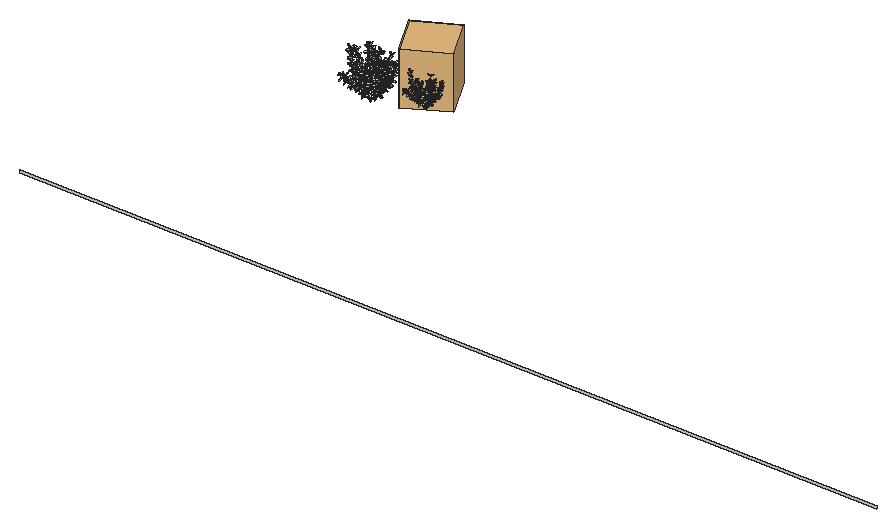
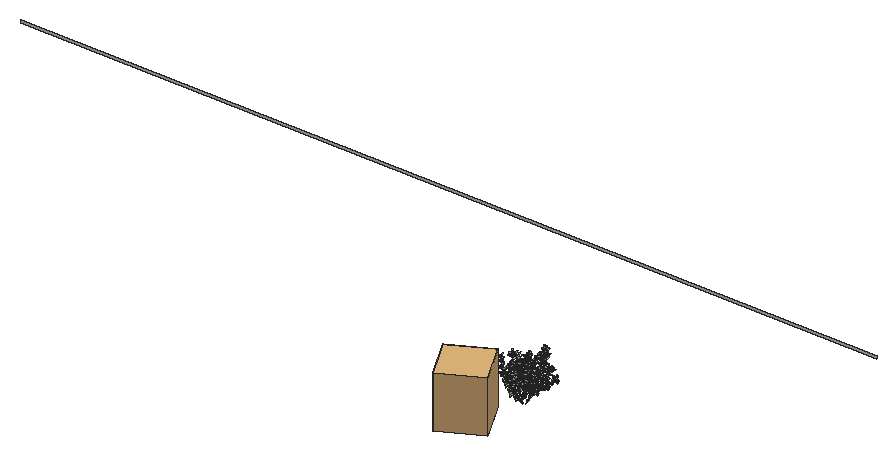
# SketchUp Ruby script. Lengths in inches.
U = 1.inch
M = Sketchup.active_model
def pt(a) = Geom::Point3d.new(a.map { |v| v * U })
def face(e, loops, mat)
  f = e.add_face(loops[0].map { |a| pt(a) })
  loops[1..].each { |l| e.add_face(l.map { |a| pt(a) }).erase! }
  f.material = f.back_material = mat if mat
  f
end
# faces: each face lists its corners as indices into pts; further lists are holes
def faces(e, pts, list, mat = nil) = list.each { |f| face(e, (f[0].is_a?(Array) ? f : [f]).map { |l| l.map { |i| pts[i] } }, mat) }
# xy, xz, yz: faces in a plane at the given z, y or x. An outline is a flat list of corners, or four numbers for a rectangle; further outlines are holes
def ring(l) = l.size == 4 ? [[l[0], l[1]], [l[2], l[1]], [l[2], l[3]], [l[0], l[3]]] : l.each_slice(2).to_a
def flat(e, list, mat, &to3) = list.each { |f| face(e, (f[0].is_a?(Array) ? f : [f]).map { |l| ring(l).map { |u, v| to3.(u, v) } }, mat) }
def xy(e, z, list, mat = nil) = flat(e, list, mat) { |x, y| [x, y, z] }
def xz(e, y, list, mat = nil) = flat(e, list, mat) { |x, z| [x, y, z] }
def yz(e, x, list, mat = nil) = flat(e, list, mat) { |y, z| [x, y, z] }
def lines(e, pts, list) = list.each { |a, b| e.add_line(pt(pts[a]), pt(pts[b])) }
# prism: a flat outline (further loops are holes) pulled along v
def prism(e, loops, v, mat = nil)
  f = face(e, loops, mat); d = Geom::Vector3d.new(v.map { |x| x * U })
  f.pushpull(f.normal.samedirection?(d) ? d.length : -d.length)
end
def box(e, o, s, mat = nil) = prism(e, [[o, [o[0] + s[0], o[1], o[2]], [o[0] + s[0], o[1] + s[1], o[2]], [o[0], o[1] + s[1], o[2]]]], [0, 0, s[2]], mat)
def at(x, y, z, deg = 0) = Geom::Transformation.translation(pt([x, y, z])) * Geom::Transformation.rotation(ORIGIN, Z_AXIS, deg.degrees)
def axes(o, x, y, z) = Geom::Transformation.new([*x, 0, *y, 0, *z, 0, *pt(o).to_a, 1])
def part(name) = M.definitions.add(name)
# library, detail: a bought-in or finely detailed component or shape, given as its bounding box
def library(name, o, s) = part(name).tap { |d| box(d.entities, o, s) }
def detail(e, o, s) = box(e.add_group.entities, o, s)
def put(e, d, t, mat = nil) = e.add_instance(d, t).tap { |i| i.material = mat if mat }
def group(e, t, mat = nil) = e.add_group.tap { |g| g.transformation = t; g.material = mat if mat }.entities
root = M.entities
M.materials.add("0ad16as01f6asdLeafVar1sfd015as60f1as6").color = [231, 235, 211]
M.materials.add("asdfasdf0165f6asdLeafVar1sfd015as60f1as6").color = [231, 235, 211]
M.materials.add("dw_stemssadfasdfa0sdf1s01d6w1").color = [90, 97, 50]
c1 = part("vdw_leaf\#1")
p = [[0,0,0],[-2.77,1.61,2.32],[-4.3125,6.1,4.5],[-3.97,13.49,6.09],[-2.47,18.57,6.3],[-0.2,22.73,5.75],
  [2.54,19.66,6.85],[4.3,15.93,7.09],[5.03,7.6,5.43],[3.32,1.76,2.74]]
faces(c1.entities,p,[[0,1,2,3,4,5],[0,5,6,7,8,9]],"0ad16as01f6asdLeafVar1sfd015as60f1as6")
c2 = part("dw_branch_3\#2")
p = [[-10.06,-1.6,62.9],[-0.2,1.54,-0.01],[-10.43,1.54,62.72],[0.18,-1.6,0.17],[-23.75,-21.66,88.91],[-25.7,-20.3,89.55],
  [13.4,11.62,104.56],[13.33,13.52,104.47],[-49.25,-41.87,130.3125],[-50.33,-40.21,130.71],[-4.97,21.13,143.98],[35.61,27.99,178.64],
  [-5.09,23.64,143.96],[35.32,29.14,178.46],[-67.7,-55.38,181.06],[-68.34,-54.45,181.62],[-22.8125,33.9,200.59],[-22.94,35.79,200.41],
  [56.61,36.78,229.75],[56.29,38.09,229.57],[-70.63,-67.46,248.85],[-70.72,-66.33,249.5],[-25.05,43.32,240.75],[-24.98,44.26,240.57]]
faces(c2.entities,p,[[0,1,2],[0,3,1],[4,2,5],[4,0,2],[6,0,2],[6,2,7],[8,4,5],[8,5,9],
  [10,6,7],[11,6,7],[10,7,12],[11,7,13],[14,8,9],[14,9,15],[16,10,12],[16,12,17],
  [18,11,13],[18,13,19],[20,14,15],[20,15,21],[22,16,17],[22,17,23]],"dw_stemssadfasdfa0sdf1s01d6w1")
c3 = part("dw_branch3\#2")
put(c3.entities,c1,axes([-70.33,-63.58,233.32],[-1.00752,0.412,0.78596],[-0.24851,-1.22189,0.32195],[0.83141,0.09817,1.01433]))
put(c3.entities,c1,axes([-66.93,-54.91,182.82],[-0.84976,-0.98359,0.33619],[0.99572,-0.74889,0.32577],[-0.05223,0.46521,1.22907]))
put(c3.entities,c1,axes([-46.12,-39.49,126.35],[1.23843,0.5364,0.23552],[-0.56438,0.94474,0.81599],[0.15707,-0.83465,1.07498]))
put(c3.entities,c1,axes([13.0625,13.13,104.77],[-1.01271,0.69982,-0.26884],[-0.74268,-0.99813,0.19939],[-0.10222,0.31872,1.21473]))
put(c3.entities,c1,axes([-18.87,30.42,186.42],[0.36309,1.06515,-0.56675],[-1.14134,0.49515,0.19939],[0.39128,0.45593,1.10754]))
put(c3.entities,c1,axes([-3.2,4.15,75.77],[-1.04153,0.55414,0.44243],[-0.23365,-1.01045,0.71554],[0.6695,0.50943,0.93801]))
put(c3.entities,c1,axes([23.2,19.41,136.3],[-0.65687,-1.11295,-0.05714],[1.05857,-0.61429,-0.20411],[0.15163,-0.1536,1.24868]))
put(c3.entities,c1,axes([-25.57,35.48,201.32],[-0.64726,0.62827,0.87973],[-0.71635,-1.0172,0.19939],[0.80962,-0.39773,0.87973]))
put(c3.entities,c1,axes([-36.37,-32.14,110.35],[-0.80747,1.09962,0.12544],[-0.83333,-0.50188,-0.96467],[-0.72833,-0.64487,0.96467]))
put(c3.entities,c1,axes([-9.89,26.72,156.79],[0.45529,1.02969,0.56572],[-1.16919,0.33753,0.32662],[0.11537,-0.64297,1.07744]))
put(c3.entities,c1,axes([-26.57,46.1,241.0625],[0.00015,0.80921,0.22536],[-0.83985,0.00446,-0.01542],[-0.01605,-0.22532,0.80906]))
put(c3.entities,c1,axes([-9.2,-2.58,61.06],[-1.10001,-0.40312,0.39014],[0.40883,-1.1116,0.00411],[0.35732,0.13566,1.14763]))
put(c3.entities,c1,axes([-69.91,-63.11,233.93],[1.36249,-0.1432,0],[0.13201,1.25603,0.5309],[-0.05549,-0.52799,1.26295]))
put(c3.entities,c1,axes([32.2,25.46,166.13],[0.06878,-1.29051,-0.05714],[1.22165,0.07415,-0.20411],[0.2113,-0.04403,1.24868]))
put(c3.entities,c1,axes([-5.68,-0.66,44.43],[-0.48448,-1.12287,0.17078],[0.98138,-0.33653,0.57135],[-0.48308,0.36756,1.04626]))
put(c3.entities,c1,axes([43.45,32.81,198.64],[0.5408,1.19584,0.14106],[-0.94242,0.32409,0.86557],[0.74952,-0.45533,0.98656]))
put(c3.entities,c1,axes([12.52,14.14,104.98],[1.02694,0.54888,0.41092],[-0.53566,1.05407,-0.06927],[-0.38969,-0.12321,1.13846]))
put(c3.entities,c1,axes([44.55,32.375,198.73],[-0.65687,-1.11295,-0.05714],[1.05857,-0.61429,-0.20411],[0.15163,-0.1536,1.24868]))
put(c3.entities,c1,axes([-5.67,21.17,141.44],[-1.10726,0.43603,-0.32953],[-0.49537,-1.03435,0.29588],[-0.17521,0.40597,1.12589]))
put(c3.entities,c1,axes([55.69,37.84,229.48],[0.18984,0.96334,0.18958],[-0.71996,0.0053,0.69399],[0.66755,-0.26823,0.69457]))
put(c3.entities,c1,axes([-21.52,36.85,205.2],[0.72606,-0.98817,0.14519],[0.94364,0.7084,0.10251],[-0.16885,0.05176,1.19664]))
put(c3.entities,c1,axes([-68.51,-56.35,196.07],[1.16319,0.72381,0],[-0.66725,1.0723,0.5309],[0.28049,-0.45075,1.26295]))
put(c3.entities,c2,at(0.01,-0.09,-0.02),"dw_stemssadfasdfa0sdf1s01d6w1")
put(c3.entities,c1,axes([-2.49,5.18,75.91],[0.78614,-0.90346,-0.30078],[0.86953,0.79562,-0.11715],[0.28546,-0.14014,1.16705]))
put(c3.entities,c1,axes([-23.125,-16.22,82.25],[0.32175,1.32576,0.12544],[-1.33153,0.31835,0.05068],[0.01989,-0.13382,1.3633]))
put(c3.entities,c1,axes([-23.75,41.99,230.3],[0.85958,-0.87451,0.14519],[0.66531,0.75721,0.62192],[-0.54076,-0.36226,1.01955]))
put(c3.entities,c1,axes([27.07,22.48,149.34],[0.92952,-0.64745,-0.62467],[0.50188,1.074,-0.36637],[0.71693,0.02135,1.04468]))
put(c3.entities,c1,axes([17.66,16.25,119.93],[-0.91649,0.83891,-0.3601],[-0.87434,-0.77966,0.40896],[0.0492,0.54447,1.14321]))
put(c3.entities,c1,axes([-68.37,-54.54,181.63],[0.32047,1.28399,0.35434],[-1.33153,0.31835,0.05068],[-0.03484,-0.35624,1.32241]))
put(c3.entities,c1,axes([-28.98,-27.1,96.48],[-0.8814,-0.35966,-0.98523],[0.75246,-1.11336,-0.26672],[-0.73065,-0.71272,0.91382]))
put(c3.entities,c1,axes([-15.23,28.43,172.72],[-1.21149,0.11898,0.32517],[-0.09739,-1.25259,0.09551],[0.33228,0.0667,1.21356]))
put(c3.entities,c1,axes([-17.5625,31.23,186.85],[-0.49275,-1.12287,0.14519],[0.95014,-0.33653,0.62192],[-0.53717,0.36756,1.01955]))
put(c3.entities,c1,axes([26.7,21.22,149.39],[-1.00104,0.22334,0.83093],[0.36894,-1.0402,0.72406],[0.77731,0.78134,0.72643]))
put(c3.entities,c1,axes([-31.125,-24.87,97.38],[0.75482,-0.86936,0.69068],[-0.00159,0.80023,1.00899],[-1.08766,-0.58016,0.45842]))
put(c3.entities,c1,axes([-71.21,-66.73,248.67],[0.25207,0.96771,0],[-0.8921,0.23237,0.38752],[0.375,-0.09768,0.92186]))
put(c3.entities,c1,axes([-24.11,41.05,229.55],[-1.11612,0.51924,-0.26884],[-0.56394,-1.10897,0.19939],[-0.15444,0.29694,1.21473]))
put(c3.entities,c1,axes([6.75,8.37,91.63],[-0.33418,-1.12287,0.39014],[1.13558,-0.33653,0.00411],[0.10478,0.36756,1.14763]))
put(c3.entities,c1,axes([-26,45.89,241.63],[-0.26986,-0.70824,-0.32129],[0.56818,-0.39091,0.38449],[-0.49365,-0.09775,0.63011]))
put(c3.entities,c1,axes([3.74,17.32,124.35],[0.22441,1.22913,-0.16274],[-1.07812,0.11178,-0.64246],[-0.61228,0.25367,1.07162]))
put(c3.entities,c1,axes([-5.44,22.27,140.88],[1.2203,0.00475,0.31374],[-0.097,1.20386,0.35905],[-0.29841,-0.37189,1.1663]))
put(c3.entities,c1,axes([-13.79,29.35,173.31],[0.83169,-0.90108,0.14519],[0.68877,0.73594,0.62192],[-0.55187,-0.34509,1.01955]))
put(c3.entities,c1,axes([-16.92,-7.26,72.98],[1.30647,0.30378,-0.27886],[0.07026,0.74892,1.14503],[0.40633,-1.10623,0.69861]))
put(c3.entities,c1,axes([4.8,17.55,125.22],[-0.25598,-1.17842,0.26559],[1.01553,-0.08455,0.60363],[-0.56975,0.35087,1.00767]))
put(c3.entities,c1,axes([5.3125,8.35,91.45],[0.00638,1.22913,-0.27714],[-1.16413,0.11178,0.46895],[0.48205,0.25367,1.13617]))
put(c3.entities,c1,axes([38.12,30.57,183.07],[1.12534,0.26182,-0.63833],[-0.46674,1.18829,-0.33545],[0.5081,0.51169,1.10563]))
put(c3.entities,c1,axes([-70.41,-60.38,214.47],[-0.41425,1.30587,0],[-1.20383,-0.38188,0.5309],[0.50605,0.16053,1.26295]))
put(c3.entities,c1,axes([37.03,28.75,180.67],[-1.12533,0.00102,-0.63799],[-0.00113,-1.2408,0],[-0.62497,0.00057,1.10237]))
put(c3.entities,c1,axes([30.71,25.35,165.96],[-0.1364,1.29314,0.22715],[-1.08768,-0.23921,0.70862],[0.73536,-0.11394,1.09026]))
put(c3.entities,c1,axes([-38.05,-30.84,110.67],[-0.31533,-1.27379,-0.2839],[1.018,-0.40311,0.67794],[-0.74394,-0.05723,1.08307]))
put(c3.entities,c1,axes([50.11,34.45,213.36],[-1.05669,0.74401,-0.05714],[-0.616,-0.82138,0.69675],[0.37221,0.60904,1.04705]))
put(c3.entities,c1,axes([-65.32,-58.78,200.07],[-1.14597,-0.19668,-0.6713],[0.21784,-1.26924,0],[-0.64812,-0.11124,1.139]))
put(c3.entities,c1,axes([-53.2,-43.37,143.59],[-0.72817,-1.09167,-0.2839],[0.82127,-0.72411,0.67794],[-0.71934,0.19815,1.08307]))
put(c3.entities,c1,axes([-61.1,-50.25,163.67],[-0.52887,1.19686,-0.30066],[-1.10762,-0.57104,-0.32484],[-0.42634,0.12264,1.23812]))
put(c3.entities,c1,axes([-54.12,-42.96,142.67],[0.32175,1.32576,0.12544],[-1.33153,0.31835,0.05068],[0.01989,-0.13382,1.3633]))
put(c3.entities,c1,axes([22.03,20.08,132.3],[1.17066,0.5058,-0.34078],[-0.35758,1.16671,0.50333],[0.49407,-0.35407,1.17172]))
put(c3.entities,c1,axes([-8.59,26.04,158.21],[-0.49275,-1.12287,0.14519],[0.95014,-0.33653,0.62192],[-0.53717,0.36756,1.01955]))
put(c3.entities,c1,axes([49.92,34.03,213.7],[1.24742,-0.35176,0.25024],[0.42127,1.159,-0.4708],[-0.09426,0.52477,1.20753]))
put(c3.entities,c1,axes([-70.34,-67.02,249.05],[-0.57048,-0.79684,0],[0.73827,-0.52855,0.24329],[-0.20203,0.14464,0.92729]))
put(c3.entities,c1,axes([56.04,36.81,228.63],[0.33451,-0.90845,-0.15237],[0.87636,0.33365,-0.06538],[0.11487,-0.11636,0.94597]))
put(c3.entities,c1,axes([-69.93,-60.58,214.88],[-0.45293,-0.99272,-0.78227],[1.14635,-0.58199,0.07483],[-0.40282,-0.65636,1.06615]))
put(c3.entities,c1,axes([-16.77,-8.59,72.7],[-1.22785,0.11509,0.53076],[-0.24879,-1.22495,-0.30991],[0.46742,-0.38989,1.16587]))
put(c3.entities,c1,axes([18.29,17.18,119.24],[1.19981,-0.45946,0.3029],[0.40159,1.22775,0.27158],[-0.37626,-0.1547,1.25575]))
put(c3.entities,c1,axes([-6.73,-0.68,43.74],[0.05346,1.22913,-0.27201],[-1.22696,0.11178,0.26396],[0.28163,0.25367,1.20164]))
put(c3.entities,c1,axes([-58.57,-48.42,160.98],[0.43385,-1.23789,0.39533],[1.04879,0.57965,0.66404],[-0.76727,0.09236,1.13122]))
put(c3.entities,c1,axes([-23.4,38.49,215.38],[0.06762,1.22913,-0.26884],[-1.23909,0.11178,0.19939],[0.21835,0.25367,1.21473]))
put(c3.entities,c1,axes([-22.21,-16.62,83.17],[-0.72817,-1.09167,-0.2839],[0.82127,-0.72411,0.67794],[-0.71934,0.19815,1.08307]))
put(c3.entities,c1,axes([-45.7,-40.77,126.53],[-1.33715,-0.0713,-0.0976],[0.07167,-1.28508,-0.04314],[-0.09306,-0.0492,1.31098]))
put(c3.entities,c1,axes([-22.39,38.51,216.12],[-0.49275,-1.12287,0.14519],[0.95014,-0.33653,0.62192],[-0.53717,0.36756,1.01955]))
c4 = part("vdw_leaf\#3")
p = [[0,0,0],[-2.77,1.61,2.32],[-4.3125,6.1,4.5],[-3.97,13.49,6.09],[-2.47,18.57,6.3],[-0.2,22.73,5.75],
  [2.54,19.66,6.85],[4.3,15.93,7.09],[5.03,7.6,5.43],[3.32,1.76,2.74]]
faces(c4.entities,p,[[0,1,2,3,4,5],[0,5,6,7,8,9]],"asdfasdf0165f6asdLeafVar1sfd015as60f1as6")
c5 = part("dw_brancj_2\#2")
p = [[9.7,-0.22,29.95],[0.23,-1.96,0.34],[-0.05,1.51,0.11],[9.65,1.51,29.46],[18.64,-8.75,84.43],[18.96,-6.63,84.625],
  [1.53,6.02,63.68],[1.42,8.18,63.25],[-10.58,8.77,161.17],[-10.41,9.98,160.68],[26.34,-9.37,211.72],[26.57,-8.28,211.23]]
faces(c5.entities,p,[[0,1,2],[0,2,3],[4,0,3],[4,3,5],[6,0,3],[6,3,7],[8,6,7],[8,7,9],
  [10,4,5],[10,5,11]],"dw_stemssadfasdfa0sdf1s01d6w1")
c6 = part("vdw_branch2\#3")
put(c6.entities,c4,axes([19.53,-5.9,102.42],[1.12377,-0.50004,0],[0.46097,1.03596,0.47664],[-0.19377,-0.43548,1.13389]))
put(c6.entities,c4,axes([-5.89,6.52,109.44],[-1.07209,0.83679,0],[-0.77141,-0.98832,0.52702],[0.32427,0.41545,1.25373]))
put(c6.entities,c4,axes([-0.44,8.23,75.28],[0.88709,-0.9947,0],[0.92159,0.82189,0.33087],[-0.25219,-0.22491,1.26111]))
put(c6.entities,c4,axes([24.71,-8.97,190.81],[-0.82641,0.91101,0],[-0.83983,-0.76184,0.47664],[0.35303,0.32025,1.13389]))
put(c6.entities,c4,axes([-2.29,8.24,91.35],[1.24603,-0.47303,0],[0.43826,1.15445,0.33087],[-0.11993,-0.31592,1.26111]))
put(c6.entities,c4,axes([12.26,-3.11,37.92],[-0.64625,1.02205,0.22511],[-1.04383,-0.61044,-0.22511],[-0.07533,-0.30931,1.18809]))
put(c6.entities,c4,axes([26.17,-9.17,210.27],[-0.99452,-0.10453,0],[0.09636,-0.91681,0.38752],[-0.04051,0.38539,0.92186]))
put(c6.entities,c4,axes([-6.07,9.4,125.35],[-0.90214,-0.98107,0],[0.90896,-0.83583,0.33087],[-0.24874,0.22873,1.26111]))
put(c6.entities,c4,axes([-4.13,7.29,110.58],[0.44715,-1.078,0.64369],[1.05816,0.63649,0.33087],[-0.58725,0.40856,1.09216]))
put(c6.entities,c4,axes([23.91,-8.22,171.96],[0.62307,0.85009,-0.63406],[-0.71531,0.8798,0.47664],[0.78296,0.12729,0.94004]))
put(c6.entities,c5,at(-0.09,0.18,-0.25),"dw_stemssadfasdfa0sdf1s01d6w1")
put(c6.entities,c4,axes([23.34,-9.65,156.59],[-0.31364,-1.00782,0.58216],[1.10369,-0.17062,0.29925],[-0.17137,0.6239,0.98776]))
put(c6.entities,c4,axes([15.03,-3.37,58.83],[-1.05425,-0.00194,0.58442],[-0.14303,-1.11707,-0.26172],[0.55355,-0.3046,0.99755]))
put(c6.entities,c4,axes([-11.625,9.46,160.37],[0.36812,0.92978,0],[-0.85713,0.33936,0.38752],[0.3603,-0.14265,0.92186]))
put(c6.entities,c4,axes([21.32,-8.53,138.72],[1.21379,0.19904,0],[-0.19904,1.21379,0],[0,0,1.23]))
put(c6.entities,c4,axes([22.54,-9.2,141.43],[-1.02887,0.17955,0.60182],[-0.23387,-1.13057,-0.06253],[0.56696,-0.17376,1.02111]))
put(c6.entities,c4,axes([23.9,-8.82,173.84],[-1.14567,-0.37474,0],[0.35918,-1.0981,0.04438],[-0.01409,0.04308,1.17993]))
put(c6.entities,c4,axes([-7.84,8.92,143.59],[-1.26971,0.40522,0],[-0.37543,-1.17638,0.33087],[0.10274,0.32192,1.26111]))
put(c6.entities,c4,axes([19.77,-8.01,85.98],[-0.32405,-1.14591,0.18674],[1.10278,-0.32969,-0.10948],[0.15845,0.14442,1.16117]))
put(c6.entities,c4,axes([-0.62,5.76,76.34],[-0.08879,1.17576,-0.67771],[-1.34525,-0.16582,-0.11144],[-0.17897,0.66309,1.17383]))
put(c6.entities,c4,axes([20.49,-8.22,121.07],[0.39924,-0.78471,-0.8233],[1.08735,0.33121,0.2116],[0.09035,-0.83005,0.83495]))
put(c6.entities,c4,axes([15.15,-3.72,62.9],[1.16251,0.40128,-0.0211],[-0.39924,1.16074,0.07874],[0.0456,-0.06757,1.2273]))
put(c6.entities,c4,axes([20.72,-8.08,120.26],[-0.03693,1.2277,-0.06551],[-1.22944,-0.03698,0],[-0.00197,0.06548,1.22825]))
put(c6.entities,c4,axes([22.58,-8.36,155.57],[-0.56247,1.09386,0],[-1.00839,-0.51852,0.47664],[0.42389,0.21796,1.13389]))
put(c6.entities,c4,axes([3.97,3.13,57.96],[-1.09459,0.76041,0],[-0.72262,-1.0402,-0.1735],[-0.10109,-0.14552,1.29352]))
put(c6.entities,c4,axes([-10.8,9.06,160.75],[-0.66334,-0.72138,0],[0.66835,-0.61458,0.24329],[-0.1829,0.16818,0.92729]))
put(c6.entities,c4,axes([19.06,-9.3125,103.96],[-1.01345,0.25553,-0.60051],[-0.2265,-1.12952,-0.09839],[-0.59598,0.03076,1.01889]))
put(c6.entities,c4,axes([18.07,-6.2,81.7],[-0.56247,1.09386,0],[-1.00839,-0.51852,0.47664],[0.42389,0.21796,1.13389]))
put(c6.entities,c4,axes([12.95,-0.39,43.31],[0.13044,-1.19832,0],[1.11025,0.12085,0.29925],[-0.30382,-0.03307,1.14057]))
put(c6.entities,c4,axes([2.28,8.28,56.18],[1.32413,-0.31027,0],[0.30923,1.31968,-0.11144],[0.02542,0.1085,1.35543]))
put(c6.entities,c4,axes([-7.55,9.96,143.07],[1.34251,-0.21744,0],[0.20045,1.23761,0.52702],[-0.08426,-0.52024,1.25373]))
put(c6.entities,c4,axes([26.15,-8.25,210.66],[0.94661,-0.25364,0],[0.235,0.87703,0.24329],[-0.06431,-0.24,0.92729]))
put(c6.entities,c4,axes([-6.48,11.37,125.16],[0.64635,1.10315,0.46356],[-1.16569,0.46153,0.52702],[0.27017,-0.6478,1.16488]))
put(c6.entities,c4,axes([25.74,-8.35,191.28],[0.13044,-1.19832,0],[1.11025,0.12085,0.29925],[-0.30382,-0.03307,1.14057]))
put(c6.entities,c4,axes([-5.125,7.47,91.6],[-1.10024,0.63688,0.48318],[-0.78682,-1.00808,-0.46292],[0.14137,-0.65404,1.184]))
c7 = part("vdw_leaf\#2")
p = [[0,0,0],[-2.77,1.61,2.32],[-4.3125,6.1,4.5],[-3.97,13.49,6.09],[-2.47,18.57,6.3],[-0.2,22.73,5.75],
  [2.54,19.66,6.85],[4.3,15.93,7.09],[5.03,7.6,5.43],[3.32,1.76,2.74]]
faces(c7.entities,p,[[0,1,2,3,4,5],[0,5,6,7,8,9]],"asdfasdf0165f6asdLeafVar1sfd015as60f1as6")
c8 = part("dg_branch_1\#2")
p = [[46.12,1.57,35.62],[46,5.42,35.41],[0.14,1.79,0.05],[0.26,-2.0625,0.27],[74.05,2.99,75.8],[74.11,5.28,75.58],
  [103.46,0.47,94.74],[104.03,2.92,94.84],[81.14,16.92,120.46],[81.2,18.78,120.24],[130.47,-5.6875,130.27],[130.58,-3.66,129.85],
  [80.82,34.4375,191.22],[80.64,35.93,190.9],[148.49,-14.56,203.24],[148.9,-12.8125,203.11],[81.08,37.95,226.93],[81.4,39.1,227.03],
  [157.45,-18.19,250.77],[157.7,-17.01,250.41]]
faces(c8.entities,p,[[0,1,2,3],[4,0,1],[4,1,5],[6,4,5],[6,5,7],[8,4,5],[8,5,9],[10,6,7],
  [10,7,11],[12,8,9],[12,9,13],[14,10,11],[14,11,15],[16,12,13],[16,13,17],[18,14,15],
  [18,15,19]],"dw_stemssadfasdfa0sdf1s01d6w1")
c9 = part("vdw_branch1\#3")
put(c9.entities,c7,axes([120.69,-2.42,117.31],[1.12221,-0.24063,-0.65809],[0.19207,1.24776,-0.12871],[0.65778,0.01392,1.11658]))
put(c9.entities,c7,axes([81,38.9,226.05],[0.7888,-0.58155,0],[0.48308,0.65523,0.47],[-0.28484,-0.38635,0.83138]))
put(c9.entities,c7,axes([78.08,12.69,106.05],[-1.43826,-0.02353,-0.03177],[0.0088,-1.31777,0.57755],[-0.03854,0.57714,1.31741]))
put(c9.entities,c7,axes([130.18,-4.73,130.41],[-0.38031,-1.29044,-0.11242],[1.20662,-0.31032,-0.51987],[0.47109,-0.24694,1.24081]))
put(c9.entities,c7,axes([157.08,-17.89,249.93],[-0.91355,0.40674,0],[-0.37496,-0.84216,0.38752],[0.15762,0.35401,0.92186]))
put(c9.entities,c7,axes([90.64,3.03,86.49],[0.32514,-0.85045,-0.99675],[0.69523,0.98247,-0.61148],[1.11061,-0.36604,0.67459]))
put(c9.entities,c7,axes([80.15,28.42,160.95],[-0.16039,0.95636,-1.06292],[-1.41646,0.03966,0.24943],[0.19509,1.07422,0.93709]))
put(c9.entities,c7,axes([126.74,-5.45,129.22],[-0.59819,0.96152,-0.6841],[-0.85772,0.12575,0.92675],[0.75427,0.88089,0.57856]))
put(c9.entities,c7,axes([133.22,-6.12,150.66],[-0.93823,0.76985,0.59124],[-0.47726,-1.08188,0.65135],[0.84525,0.24366,1.02405]))
put(c9.entities,c7,axes([80.43,22.89,141.32],[-1.42571,-0.19312,0.01373],[0.18338,-1.31425,0.5561],[-0.0621,0.5528,1.32692]))
put(c9.entities,c7,axes([33.14,0.88,26.42],[-0.13338,1.31536,0.04876],[-1.04528,-0.13221,0.7073],[0.72315,0.03348,1.07497]))
put(c9.entities,c7,axes([152.63,-15.08,221.76],[-1.28188,0.41945,0.0579],[-0.3638,-1.18547,0.53367],[0.21665,0.49113,1.23869]))
put(c9.entities,c7,axes([80.05,28.28,160.33],[-0.46732,-1.26661,0.40679],[1.27397,-0.40257,0.21004],[-0.07408,0.44645,1.30501]))
put(c9.entities,c7,axes([153.95,-14.8,235.875],[0.39005,1.07743,0.20605],[-0.96443,0.25296,0.50293],[0.42961,-0.3464,0.99807]))
put(c9.entities,c7,axes([80.2,24.22,141.74],[1.33062,-0.46576,0.02628],[0.44746,1.2746,-0.06608],[-0.00197,0.0722,1.37936]))
put(c9.entities,c7,axes([145.48,-12.5,188.92],[-1.32952,0.16983,0.16138],[-0.09299,-1.2361,0.53471],[0.21503,0.51548,1.22904]))
put(c9.entities,c7,axes([139.64,-9.18,171.24],[0.05682,1.30088,0.23414],[-1.13176,-0.05343,0.57151],[0.58357,-0.22963,1.13417]))
put(c9.entities,c7,axes([70.95,4.35,71.98],[-1.1081,-0.41873,0.64752],[0.33675,-1.28259,-0.25313],[0.6937,-0.04625,1.15721]))
put(c9.entities,c7,axes([59.85,4.55,56.17],[-0.26797,1.24526,0.35754],[-0.9369,-0.41634,0.74783],[0.83377,-0.10389,0.98674]))
put(c9.entities,c7,axes([33.11,3.36,25.66],[-0.57817,-1.07968,-0.5679],[1.11554,-0.21356,-0.7297],[0.49375,-0.78178,0.98363]))
put(c9.entities,c8,at(-0.21,0.34,-0.17),"dw_stemssadfasdfa0sdf1s01d6w1")
put(c9.entities,c7,axes([80.91,19.01,122.53],[-0.84258,1.13222,-0.27981],[-1.15093,-0.75138,0.42537],[0.18861,0.47293,1.3457]))
put(c9.entities,c7,axes([119.8,-1.22,114.1],[-1.3235,-0.25012,0.09101],[0.25933,-1.31572,0.15537],[0.05991,0.1698,1.33794]))
put(c9.entities,c7,axes([46.29,5.1,38.04],[0.98937,0.73827,-0.47585],[-0.72359,1.03721,0.10473],[0.44068,0.18581,1.20453]))
put(c9.entities,c7,axes([81.1875,33.03,184.45],[1.33883,0.26986,0.35053],[-0.09581,1.22087,-0.57399],[-0.42216,0.53228,1.20262]))
put(c9.entities,c7,axes([80.16,36.28,206.98],[-0.83993,0.85737,-0.6234],[-1.05964,-0.65701,0.5241],[0.02941,0.81391,1.07976]))
put(c9.entities,c7,axes([154.86,-16.15,234.87],[0.02509,-1.15302,-0.28506],[1.1487,-0.04894,0.29908],[-0.30202,-0.28195,1.11384]))
put(c9.entities,c7,axes([108.77,-0.33,101.14],[-0.47691,-1.03266,-0.72709],[1.25395,-0.29455,-0.40416],[0.15052,-0.81814,1.06325]))
put(c9.entities,c7,axes([89.79,3.01,85.87],[-0.61344,0.75518,0.8965],[-0.17758,-1.01824,0.73622],[1.13385,0.22574,0.58569]))
put(c9.entities,c7,axes([81.56,20.31,123.29],[0.37259,-1.3435,0.21057],[1.29385,0.32364,-0.22445],[0.16906,0.25791,1.34638]))
put(c9.entities,c7,axes([46.45,1.82,36.74],[-0.77883,0.29892,1.0614],[0.19124,-1.24314,0.49044],[1.08598,0.43329,0.67484]))
put(c9.entities,c7,axes([71.37,4.02,72.32],[0.72905,0.81546,-0.74421],[-0.66805,0.98958,0.42988],[0.8391,0.14186,0.97745]))
put(c9.entities,c7,axes([136.59,-5.88,150.53],[0.85845,-0.99897,-0.12437],[0.96526,0.81273,0.13453],[-0.02572,-0.18182,1.28292]))
put(c9.entities,c7,axes([80.375,38.8,225.86],[-0.25178,0.96778,0],[-0.89216,-0.23211,0.38752],[0.37503,0.09757,0.92186]))
put(c9.entities,c7,axes([74.43,7.99,85.38],[-1.05703,0.91669,-0.33543],[-0.95806,-0.87958,0.61531],[0.18697,0.6754,1.25659]))
put(c9.entities,c7,axes([76.57,9.74,89.32],[0.63146,-1.21538,0.33508],[1.18148,0.49387,-0.43517],[0.26321,0.48577,1.26593]))
put(c9.entities,c7,axes([81.6875,36.97,207.4],[0.09422,-1.04424,0.38486],[1.01646,0.1939,0.27727],[-0.33299,0.33382,0.98727]))
put(c9.entities,c7,axes([157.29,-17.17,249.98],[0.50586,-0.50586,0],[0.38853,0.38853,0.41105],[-0.29684,-0.29684,0.56115]))
put(c9.entities,c7,axes([79.92,15.8,106.09],[1.03917,-0.29343,-0.90675],[-0.14587,1.22131,-0.5624],[0.92163,0.5191,0.88824]))
put(c9.entities,c7,axes([61.95,3.88,56.26],[0.41243,-1.28546,0],[1.17466,0.37688,-0.54831],[0.5221,0.16751,1.23363]))
put(c9.entities,c7,axes([151.99,-14.79,208.15],[-0.48571,-1.21723,-0.32393],[1.25386,-0.50033,0],[-0.12005,-0.30087,1.31056]))
put(c9.entities,c7,axes([108.44,0.62,102.22],[0.82183,0.96078,0.38967],[-0.62327,0.08618,1.10203],[0.79141,-0.88661,0.51693]))
put(c9.entities,c7,axes([145.6,-10.56,188.62],[1.03241,-0.02554,-0.82693],[0.3944,1.11584,0.45794],[0.70325,-0.61672,0.89706]))
put(c9.entities,c7,axes([78.59,32.3,183.89],[-1.12675,-0.42036,0.43987],[0.5899,-0.98149,0.57312],[0.14901,0.70693,1.05726]))
put(c9.entities,c7,axes([152.08,-13.42,223.37],[0.79993,-0.44251,-0.69938],[0.68456,0.82615,0.26026],[0.41048,-0.60953,0.85515]))
put(c9.entities,c7,axes([140.71,-8.74,170.55],[0.41903,-1.24177,-0.32393],[1.26224,0.33728,0.33986],[-0.23168,-0.40836,1.26573]))
put(c9.entities,c7,axes([149.25,-12.53,205.78],[1.24456,0.38285,0.23414],[-0.42999,1.04826,0.57151],[-0.02056,-0.62679,1.13417]))
c10 = library("Narrowleaf plant",[-0.44,-0.75,-1.28],[7.48,8.05,9.01])
xz(root,0,[[2076.625,-9,3026.5,-6]])
put(root,c3,axes([2248.24,276.4,10.58],[0.09481,-0.08589,0.04174],[0.08433,0.10034,0.02262],[-0.03765,0.00844,0.15579]))
put(root,c3,axes([2249.4375,269.98,3.93],[-0.12304,0.0546,-0.04713],[-0.02701,-0.11428,-0.0937],[-0.06098,-0.05955,0.13659]))
put(root,c3,axes([2246.83,269.36,7.47],[0.1634,0,0],[0,0.1634,0],[0,0,0.20106]))
put(root,c6,axes([2249.08,274.45,6.3],[0.0097,0.14118,-0.10053],[-0.16302,0.01121,0],[0.0056,0.08151,0.17413]))
put(root,c9,axes([2246.38,269.59,7.1875],[0.01907,-0.13922,0],[0.13922,0.01907,0],[0,0,0.17291]))
put(root,c6,axes([2253.18,270.625,5.57],[0.02729,0.1244,-0.09048],[-0.14364,0.03151,0],[0.01575,0.07182,0.15671]))
put(root,c6,axes([2248.87,269.52,5.4],[0.09858,-0.0952,-0.10951],[0.11351,0.11754,0],[0.06402,-0.06182,0.16863]))
put(root,c6,axes([2254.1,269.95,8.3],[0.15791,0.02906,-0.03733],[-0.02958,0.1607,0],[0.02984,0.00549,0.19757]))
put(root,c9,axes([2251.86,271.36,7.18],[0.11749,0.04939,0],[-0.04939,0.11749,0],[0,0,0.15683]))
put(root,c3,axes([2279.7,324,0.76],[-0.0835,0.03705,-0.03198],[-0.01833,-0.07755,-0.06358],[-0.04138,-0.04041,0.09269]))
put(root,c3,axes([2277.9375,323.58,3.17],[0.11088,0,0],[0,0.11088,0],[0,0,0.13644]))
put(root,c10,axes([2270.11,289.28,7.7],[5.63682,3.11169,0],[-3.11169,5.63682,0],[0,0,6.43866]))
put(root,c9,axes([2287.23,295.83,2.97],[-0.07583,0.05409,0],[-0.05409,-0.07583,0],[0,0,0.11461]))
put(root,c9,axes([2277.625,323.74,2.97],[0.01294,-0.09448,0],[0.09448,0.01294,0],[0,0,0.11734]))
put(root,c6,axes([2285.17,294.97,3.23],[-0.06851,-0.04024,-0.04853],[0.04493,-0.07649,0],[-0.03401,-0.01998,0.09777]))
put(root,c6,axes([2285.08,295.88,3.73],[-0.10632,-0.02382,-0.02533],[0.02424,-0.1082,0],[-0.02009,-0.0045,0.13407]))
put(root,c3,axes([2289.18,298.52,5.28],[0.06434,-0.05829,0.02833],[0.05722,0.06809,0.01535],[-0.02555,0.00573,0.10572]))
put(root,c6,axes([2279.31,323.6875,1.76],[0.06689,-0.0646,-0.07431],[0.07703,0.07976,0],[0.04344,-0.04195,0.11443]))
put(root,c3,axes([2289.99,294.17,0.76],[-0.0835,0.03705,-0.03198],[-0.01833,-0.07755,-0.06358],[-0.04138,-0.04041,0.09269]))
put(root,c3,axes([2288.23,293.75,3.17],[0.11088,0,0],[0,0.11088,0],[0,0,0.13644]))
put(root,c6,axes([2289.75,297.2,2.375],[0.00659,0.0958,-0.06822],[-0.11062,0.0076,0],[0.0038,0.05531,0.11816]))
put(root,c9,axes([2287.92,293.9,2.97],[0.01294,-0.09448,0],[0.09448,0.01294,0],[0,0,0.11734]))
put(root,c6,axes([2292.54,294.61,1.88],[0.01852,0.08442,-0.0614],[-0.09748,0.02138,0],[0.01069,0.04874,0.10635]))
put(root,c6,axes([2289.61,293.85,1.76],[0.06689,-0.0646,-0.07431],[0.07703,0.07976,0],[0.04344,-0.04195,0.11443]))
put(root,c6,axes([2293.16,294.15,3.73],[0.10716,0.01972,-0.02533],[-0.02007,0.10905,0],[0.02025,0.00373,0.13407]))
put(root,c9,axes([2291.64,295.1,2.97],[0.07973,0.03352,0],[-0.03352,0.07973,0],[0,0,0.10642]))
